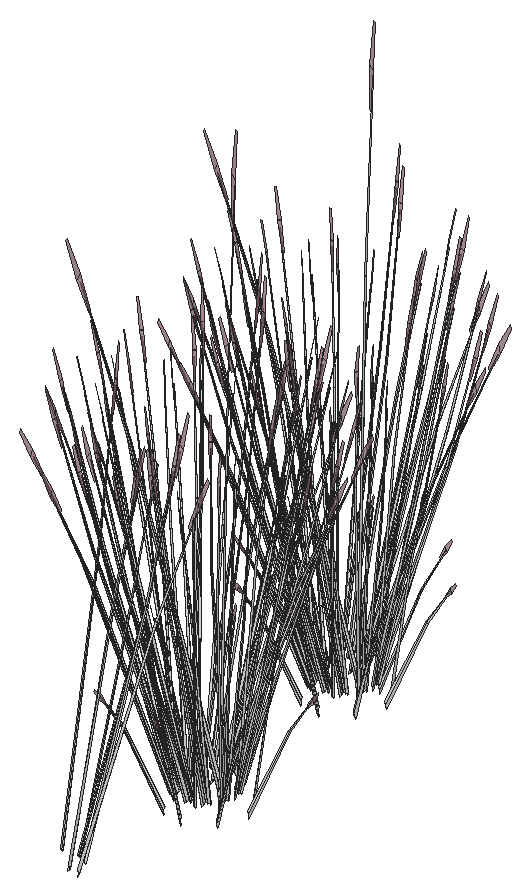
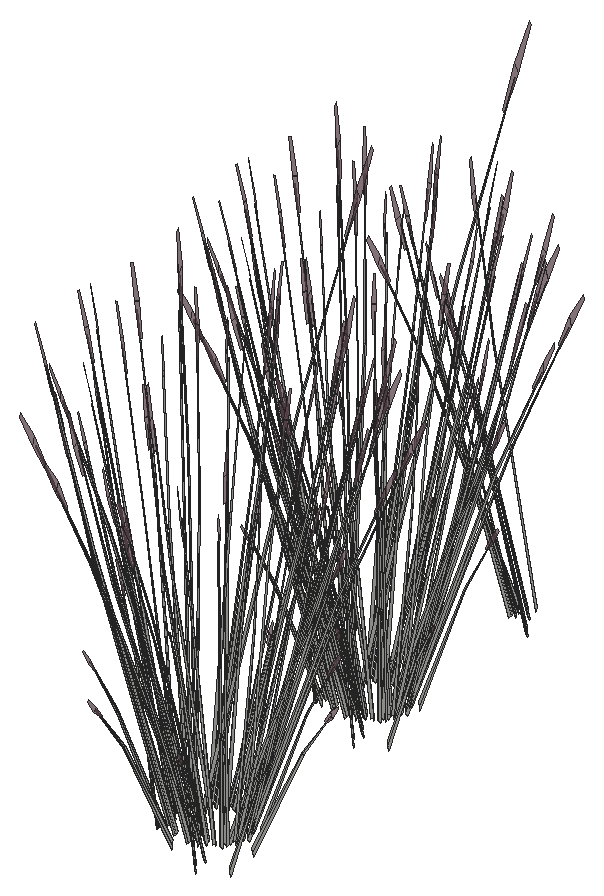
# SketchUp Ruby script. Lengths in inches.
U = 1.inch
M = Sketchup.active_model
def pt(a) = Geom::Point3d.new(a.map { |v| v * U })
def face(e, loops, mat)
  f = e.add_face(loops[0].map { |a| pt(a) })
  loops[1..].each { |l| e.add_face(l.map { |a| pt(a) }).erase! }
  f.material = f.back_material = mat if mat
  f
end
# faces: each face lists its corners as indices into pts; further lists are holes
def faces(e, pts, list, mat = nil) = list.each { |f| face(e, (f[0].is_a?(Array) ? f : [f]).map { |l| l.map { |i| pts[i] } }, mat) }
# xy, xz, yz: faces in a plane at the given z, y or x. An outline is a flat list of corners, or four numbers for a rectangle; further outlines are holes
def ring(l) = l.size == 4 ? [[l[0], l[1]], [l[2], l[1]], [l[2], l[3]], [l[0], l[3]]] : l.each_slice(2).to_a
def flat(e, list, mat, &to3) = list.each { |f| face(e, (f[0].is_a?(Array) ? f : [f]).map { |l| ring(l).map { |u, v| to3.(u, v) } }, mat) }
def xy(e, z, list, mat = nil) = flat(e, list, mat) { |x, y| [x, y, z] }
def xz(e, y, list, mat = nil) = flat(e, list, mat) { |x, z| [x, y, z] }
def yz(e, x, list, mat = nil) = flat(e, list, mat) { |y, z| [x, y, z] }
def lines(e, pts, list) = list.each { |a, b| e.add_line(pt(pts[a]), pt(pts[b])) }
# prism: a flat outline (further loops are holes) pulled along v
def prism(e, loops, v, mat = nil)
  f = face(e, loops, mat); d = Geom::Vector3d.new(v.map { |x| x * U })
  f.pushpull(f.normal.samedirection?(d) ? d.length : -d.length)
end
def box(e, o, s, mat = nil) = prism(e, [[o, [o[0] + s[0], o[1], o[2]], [o[0] + s[0], o[1] + s[1], o[2]], [o[0], o[1] + s[1], o[2]]]], [0, 0, s[2]], mat)
def at(x, y, z, deg = 0) = Geom::Transformation.translation(pt([x, y, z])) * Geom::Transformation.rotation(ORIGIN, Z_AXIS, deg.degrees)
def axes(o, x, y, z) = Geom::Transformation.new([*x, 0, *y, 0, *z, 0, *pt(o).to_a, 1])
def part(name) = M.definitions.add(name)
# library, detail: a bought-in or finely detailed component or shape, given as its bounding box
def library(name, o, s) = part(name).tap { |d| box(d.entities, o, s) }
def detail(e, o, s) = box(e.add_group.entities, o, s)
def put(e, d, t, mat = nil) = e.add_instance(d, t).tap { |i| i.material = mat if mat }
def group(e, t, mat = nil) = e.add_group.tap { |g| g.transformation = t; g.material = mat if mat }.entities
root = M.entities
M.materials.add("LightPink_Translucent").color = [144, 107, 117]
M.materials["LightPink_Translucent"].alpha = 0.75
c1 = part("blade")
p = [[2.15,0.21,22],[0,0.17,0],[0.09,0.45,0],[2.18,0.31,22],[2.29,0.31,22],[0.38,0.45,0],
  [2.48,0.24,33],[2.49,0.24,33],[2.48,0.22,33]]
faces(c1.entities,p,[[0,1,2,3],[4,5,2,3],[6,3,4,7],[8,0,3,6]])
c2 = part("seeds")
p = [[0.3,-0.1,1.38],[-0.01,-0.03,1.59],[-0.01,-0.03,0.03],[0.14,-0.07,-0.07],[0.29,-0.03,3],[0.15,0.01,3.11]]
faces(c2.entities,p,[[0,1,2,3],[1,0,4,5]],"LightPink_Translucent")
c3 = part("blade with seeds")
put(c3.entities,c1,at(0,0,0))
put(c3.entities,c2,axes([2.4,0.25,30.99],[1.5799,-0.05474,1.17369],[-0.12525,1.92788,0.29478],[-0.07173,-0.02425,1.56792]))
put(root,c3,axes([335.52,111.16,268.36],[0.50273,0.13626,-0.47583],[-0.17232,0.46717,-0.36857],[0.0461,0.18809,0.91046]))
put(root,c3,axes([335.81,110.19,267.61],[-0.1169,-0.17452,1.59586],[0.54019,-0.14692,0.12904],[0.12209,0.27397,0.68222]))
put(root,c3,axes([335.29,111.45,268.22],[-0.15418,0.41799,-0.32977],[-0.44981,-0.12192,0.42575],[0.04124,0.16829,0.81462]))
put(root,c3,axes([334.32,110.64,268.97],[-0.01331,0.50278,-0.73435],[-0.56035,-0.03377,0.08862],[-0.05914,0.213,1.03881]))
put(root,c3,axes([334.85,110.28,267.61],[-0.01252,-0.20862,1.59586],[0.54251,0.1384,0.12904],[-0.03356,0.2973,0.68222]))
put(root,c3,axes([335.34,111.07,268.64],[0.24409,0.44196,-0.66157],[-0.50245,0.2463,0.07984],[0.05708,0.21354,0.93586]))
put(root,c3,axes([334.13,111.35,267.13],[0.01124,-0.2806,1.43727],[0.50537,0.14821,0.19862],[-0.04379,0.29905,0.67868]))
put(root,c3,axes([334.52,122.62,267.61],[0.1169,0.17452,1.59586],[-0.54019,0.14692,0.12904],[-0.12209,-0.27397,0.68222]))
put(root,c3,axes([335.96,122.75,268.64],[-0.24409,-0.44196,-0.66157],[0.50245,-0.2463,0.07984],[-0.05708,-0.21354,0.93586]))
put(root,c3,axes([336.98,123.18,268.64],[0.01331,-0.50278,-0.66157],[0.56035,0.03377,0.07984],[0.05914,-0.213,0.93586]))
put(root,c3,axes([336.01,122.37,268.22],[0.15418,-0.41799,-0.32977],[0.44981,0.12192,0.42575],[-0.04124,-0.16829,0.81462]))
put(root,c3,axes([336.35,122.92,267.61],[-0.09522,0.18683,1.59586],[-0.39947,-0.38663,0.12904],[0.18021,-0.24097,0.68222]))
put(root,c3,axes([335.78,122.66,268.36],[-0.50273,-0.13626,-0.47583],[0.17232,-0.46717,-0.36857],[-0.0461,-0.18809,0.91046]))
put(root,c3,axes([336.09,121.49,266.58],[0.06561,0.31695,1.06958],[-0.36394,-0.17555,0.78586],[0.03916,-0.16229,0.23558]))
put(root,c3,axes([336.86,123.01,268.36],[-0.3661,-0.36521,-0.47583],[0.38674,-0.31985,-0.36857],[0.0557,-0.18556,0.91046]))
put(root,c3,axes([336.21,122.64,268.6875],[-0.50045,0.25306,-0.11324],[-0.24593,-0.44915,-0.62851],[-0.06603,-0.18927,0.95501]))
put(root,c3,axes([337.25,123.2,268.6875],[-0.56206,-0.02693,-0.11324],[0.01536,-0.50991,-0.62851],[0.03904,-0.19638,0.95501]))
put(root,c3,axes([337.21,122.88,268.22],[0.34603,-0.28618,-0.32977],[0.32756,0.32677,0.42575],[0.04984,-0.16603,0.81462]))
put(root,c3,axes([334.22,121.87,266.58],[0.26677,0.18918,1.06958],[-0.38851,0.11372,0.78586],[-0.08313,-0.14539,0.23558]))
put(root,c3,axes([334.86,122.87,268.64],[-0.43608,-0.26272,-0.66157],[0.30991,-0.46038,0.07984],[-0.158,-0.15687,0.93586]))
put(root,c3,axes([334.71,122.53,268.22],[-0.07899,-0.43781,-0.32977],[0.45153,-0.11561,0.42575],[-0.12128,-0.12546,0.81462]))
put(root,c3,axes([333.74,123.16,267.61],[0.18996,0.09365,1.59586],[-0.39312,0.39287,0.12904],[-0.24502,-0.17723,0.68222]))
put(root,c3,axes([334.66,122.89,268.36],[-0.50465,0.12921,-0.47583],[-0.08828,-0.48932,-0.36857],[-0.13555,-0.14022,0.91046]))
put(root,c3,axes([337.64,124.05,268.64],[0.26714,-0.42887,-0.66157],[0.46811,0.30479,0.07984],[0.1595,-0.15539,0.93586]))
put(root,c3,axes([337.625,123.85,268.36],[-0.13138,-0.49631,-0.47583],[0.49754,-0.08682,-0.36857],[0.14258,-0.13331,0.91046]))
put(root,c3,axes([337.86,124.21,268.6875],[-0.47307,-0.29971,-0.11324],[0.27254,-0.43404,-0.62851],[0.13365,-0.15087,0.95501]))
put(root,c3,axes([335.91,125.85,267.1],[0.44194,0.21918,1.40854],[-0.43295,0.47219,0.557],[-0.19393,-0.27986,1.18082]))
put(root,c3,axes([338.24,122.87,266.58],[-0.17034,0.27669,1.06958],[-0.14642,-0.37174,0.78586],[0.14069,-0.09315,0.23558]))
put(root,c3,axes([337.99,123.91,268.22],[0.44516,-0.07768,-0.32977],[0.11755,0.44407,0.42575],[0.12757,-0.11927,0.81462]))
put(root,c3,axes([333.67,123.3,268.22],[-0.29098,-0.34031,-0.32977],[0.33226,-0.32215,0.42575],[-0.16881,-0.04902,0.81462]))
put(root,c3,axes([333.97,123.52,268.64],[-0.51122,-0.01309,-0.66157],[0.03434,-0.5511,0.07984],[-0.21658,-0.05816,0.93586]))
put(root,c3,axes([333.8,123.63,268.36],[-0.37135,0.36005,-0.47583],[-0.32522,-0.38035,-0.36857],[-0.18868,-0.05478,0.91046]))
put(root,c3,axes([334,123.26,268.6875],[-0.02738,0.55277,-0.11324],[-0.51847,-0.01511,-0.62851],[-0.19968,-0.0384,0.95501]))
put(root,c3,axes([337.88,125.38,268.6875],[-0.25732,-0.49218,-0.11324],[0.45669,-0.24187,-0.62851],[0.19245,-0.06494,0.95501]))
put(root,c3,axes([337.86,124.96,268.36],[0.13855,-0.49442,-0.47583],[0.47502,0.16947,-0.36857],[0.19125,-0.04534,0.91046]))
put(root,c3,axes([333.34,124.02,267.61],[0.21212,-0.01231,1.59586],[-0.14072,0.53355,0.12904],[-0.3023,-0.033,0.68222]))
put(root,c3,axes([337.77,125.14,268.64],[0.44939,-0.24006,-0.66157],[0.25044,0.49415,0.07984],[0.21713,-0.05613,0.93586]))
put(root,c3,axes([338.15,125.18,268.22],[0.42502,0.15163,-0.32977],[-0.12396,0.44238,0.42575],[0.17112,-0.04056,0.81462]))
put(root,c3,axes([333.15,124.48,268.22],[-0.42502,-0.15163,-0.32977],[0.12396,-0.44238,0.42575],[-0.17112,0.04056,0.81462]))
put(root,c3,axes([336.99,124.63,267.61],[-0.21212,0.01231,1.59586],[0.14072,-0.53355,0.12904],[0.3023,0.033,0.68222]))
put(root,c3,axes([334.45,124.4,267.11],[0.14537,-0.07863,1.64882],[0.05013,0.549,0.12904],[-0.31487,0.07285,0.5893]))
put(root,c3,axes([339.05,125.27,266.58],[-0.31598,0.08973,1.06958],[0.14873,-0.37085,0.78586],[0.16763,0.02538,0.23558]))
put(root,c3,axes([333.44,124.7,268.36],[-0.13855,0.49442,-0.47583],[-0.47502,-0.16947,-0.36857],[-0.19125,0.04534,0.91046]))
put(root,c3,axes([333.42,124.28,268.6875],[0.25732,0.49218,-0.11324],[-0.45669,0.24187,-0.62851],[-0.19245,0.06494,0.95501]))
put(root,c3,axes([338.5,126.41,267.66],[-0.09788,-0.45691,-0.03251],[0.46264,-0.10504,-0.14742],[0.09661,0.02897,0.48626]))
put(root,c3,axes([337.3,126.4,268.6875],[0.02738,-0.55277,-0.11324],[0.51847,0.01511,-0.62851],[0.19968,0.0384,0.95501]))
put(root,c3,axes([333.43,124.96,267.61],[0.17745,-0.11497,1.59586],[0.14939,0.53127,0.12904],[-0.27857,0.12007,0.68222]))
put(root,c3,axes([337.33,126.14,268.64],[0.51122,0.01309,-0.66157],[-0.03434,0.5511,0.07984],[0.21658,0.05816,0.93586]))
put(root,c3,axes([332.5,126.82,266.58],[0.21313,-0.24635,1.06958],[0.0841,0.38999,0.78586],[-0.15402,0.06983,0.23558]))
put(root,c3,axes([337.63,126.36,268.22],[0.29098,0.34031,-0.32977],[-0.33226,0.32215,0.42575],[0.16881,0.04902,0.81462]))
put(root,c3,axes([333.31,125.75,268.22],[-0.44516,0.07768,-0.32977],[-0.11755,-0.44407,0.42575],[-0.12757,0.11927,0.81462]))
put(root,c3,axes([336.59,125.49,267.61],[-0.18996,-0.09365,1.59586],[0.39312,-0.39287,0.12904],[0.24502,0.17723,0.68222]))
put(root,c3,axes([333.44,125.45,268.6875],[0.47307,0.29971,-0.11324],[-0.27254,0.43404,-0.62851],[-0.13365,0.15087,0.95501]))
put(root,c3,axes([336.28,127,268.6875],[0.30474,-0.46525,-0.11324],[0.44133,0.26804,-0.62851],[0.15341,0.13145,0.95501]))
put(root,c3,axes([334.08,125.31,267.61],[0.12773,-0.16701,1.59586],[0.32252,0.4508,0.12904],[-0.22121,0.20529,0.68222]))
put(root,c3,axes([333.67,125.8,268.36],[0.13138,0.49631,-0.47583],[-0.49754,0.08682,-0.36857],[-0.14258,0.13331,0.91046]))
put(root,c3,axes([336.59,124.8,266.65],[-0.01397,-0.51177,1.31553],[0.63227,0.13266,0.557],[-0.14954,0.28003,1.24175]))
put(root,c3,axes([336.64,126.77,268.36],[0.50465,-0.12921,-0.47583],[0.08828,0.48932,-0.36857],[0.13555,0.14022,0.91046]))
put(root,c3,axes([333.98,125.73,267.61],[0.09522,-0.18683,1.59586],[0.39947,0.38663,0.12904],[-0.18021,0.24097,0.68222]))
put(root,c3,axes([334.09,126.78,268.22],[-0.34603,0.28618,-0.32977],[-0.32756,-0.32677,0.42575],[-0.04984,0.16603,0.81462]))
put(root,c3,axes([335.09,127.02,268.6875],[0.50045,-0.25306,-0.11324],[0.24593,0.44915,-0.62851],[0.06603,0.18927,0.95501]))
put(root,c3,axes([334.3125,127.89,266.58],[-0.01324,-0.32319,1.06958],[0.33072,0.23052,0.78586],[-0.06504,0.15405,0.23558]))
put(root,c3,axes([334.43,126.64,268.66],[0.3661,0.36521,-0.52818],[-0.38674,0.31985,-0.40911],[-0.0557,0.18556,1.01061]))
put(root,c3,axes([335.52,127,268.36],[0.50273,0.13626,-0.47583],[-0.17232,0.46717,-0.36857],[0.0461,0.18809,0.91046]))
put(root,c3,axes([335.81,126.03,267.61],[-0.1169,-0.17452,1.59586],[0.54019,-0.14692,0.12904],[0.12209,0.27397,0.68222]))
put(root,c3,axes([335.29,127.29,268.22],[-0.15418,0.41799,-0.32977],[-0.44981,-0.12192,0.42575],[0.04124,0.16829,0.81462]))
put(root,c3,axes([334.32,126.48,268.97],[-0.01331,0.50278,-0.73435],[-0.56035,-0.03377,0.08862],[-0.05914,0.213,1.03881]))
put(root,c3,axes([334.85,126.12,267.61],[-0.01252,-0.20862,1.59586],[0.54251,0.1384,0.12904],[-0.03356,0.2973,0.68222]))
put(root,c3,axes([335.34,126.91,268.64],[0.24409,0.44196,-0.66157],[-0.50245,0.2463,0.07984],[0.05708,0.21354,0.93586]))
put(root,c3,axes([334.13,127.1875,267.13],[0.01124,-0.2806,1.43727],[0.50537,0.14821,0.19862],[-0.04379,0.29905,0.67868]))
put(root,c3,axes([332.31,140.63,267.61],[0.1169,0.17452,1.59586],[-0.54019,0.14692,0.12904],[-0.12209,-0.27397,0.68222]))
put(root,c3,axes([333.75,140.76,268.64],[-0.24409,-0.44196,-0.66157],[0.50245,-0.2463,0.07984],[-0.05708,-0.21354,0.93586]))
put(root,c3,axes([334.76,141.19,268.64],[0.01331,-0.50278,-0.66157],[0.56035,0.03377,0.07984],[0.05914,-0.213,0.93586]))
put(root,c3,axes([333.79,140.38,268.22],[0.15418,-0.41799,-0.32977],[0.44981,0.12192,0.42575],[-0.04124,-0.16829,0.81462]))
put(root,c3,axes([334.13,140.93,267.61],[-0.09522,0.18683,1.59586],[-0.39947,-0.38663,0.12904],[0.18021,-0.24097,0.68222]))
put(root,c3,axes([333.5625,140.67,268.36],[-0.50273,-0.13626,-0.47583],[0.17232,-0.46717,-0.36857],[-0.0461,-0.18809,0.91046]))
put(root,c3,axes([333.875,139.5,266.58],[0.06561,0.31695,1.06958],[-0.36394,-0.17555,0.78586],[0.03916,-0.16229,0.23558]))
put(root,c3,axes([334.65,141.02,268.36],[-0.3661,-0.36521,-0.47583],[0.38674,-0.31985,-0.36857],[0.0557,-0.18556,0.91046]))
put(root,c3,axes([335.03,141.21,268.6875],[-0.56206,-0.02693,-0.11324],[0.01536,-0.50991,-0.62851],[0.03904,-0.19638,0.95501]))
put(root,c3,axes([334.99,140.89,268.22],[0.34603,-0.28618,-0.32977],[0.32756,0.32677,0.42575],[0.04984,-0.16603,0.81462]))
put(root,c3,axes([332,139.88,266.58],[0.26677,0.18918,1.06958],[-0.38851,0.11372,0.78586],[-0.08313,-0.14539,0.23558]))
put(root,c3,axes([332.65,140.88,268.64],[-0.43608,-0.26272,-0.66157],[0.30991,-0.46038,0.07984],[-0.158,-0.15687,0.93586]))
put(root,c3,axes([332.5,140.53,268.22],[-0.07899,-0.43781,-0.32977],[0.45153,-0.11561,0.42575],[-0.12128,-0.12546,0.81462]))
put(root,c3,axes([331.52,141.17,267.61],[0.18996,0.09365,1.59586],[-0.39312,0.39287,0.12904],[-0.24502,-0.17723,0.68222]))
put(root,c3,axes([332.44,140.9,268.36],[-0.50465,0.12921,-0.47583],[-0.08828,-0.48932,-0.36857],[-0.13555,-0.14022,0.91046]))
put(root,c3,axes([335.42,142.0625,268.64],[0.26714,-0.42887,-0.66157],[0.46811,0.30479,0.07984],[0.1595,-0.15539,0.93586]))
put(root,c3,axes([335.41,141.86,268.36],[-0.13138,-0.49631,-0.47583],[0.49754,-0.08682,-0.36857],[0.14258,-0.13331,0.91046]))
put(root,c3,axes([333.69,143.85,267.1],[0.44194,0.21918,1.40854],[-0.43295,0.47219,0.557],[-0.19393,-0.27986,1.18082]))
put(root,c3,axes([336.02,140.875,266.58],[-0.17034,0.27669,1.06958],[-0.14642,-0.37174,0.78586],[0.14069,-0.09315,0.23558]))
put(root,c3,axes([335.78,141.92,268.22],[0.44516,-0.07768,-0.32977],[0.11755,0.44407,0.42575],[0.12757,-0.11927,0.81462]))
put(root,c3,axes([331.45,141.31,268.22],[-0.29098,-0.34031,-0.32977],[0.33226,-0.32215,0.42575],[-0.16881,-0.04902,0.81462]))
put(root,c3,axes([331.76,141.53,268.64],[-0.51122,-0.01309,-0.66157],[0.03434,-0.5511,0.07984],[-0.21658,-0.05816,0.93586]))
put(root,c3,axes([331.59,141.64,268.36],[-0.37135,0.36005,-0.47583],[-0.32522,-0.38035,-0.36857],[-0.18868,-0.05478,0.91046]))
put(root,c3,axes([330.75,142.12,266.58],[0.3265,-0.03889,1.06958],[-0.20711,0.3427,0.78586],[-0.16135,-0.05141,0.23558]))
put(root,c3,axes([331.78,141.27,268.6875],[-0.02738,0.55277,-0.11324],[-0.51847,-0.01511,-0.62851],[-0.19968,-0.0384,0.95501]))
put(root,c3,axes([335.66,143.39,268.6875],[-0.25732,-0.49218,-0.11324],[0.45669,-0.24187,-0.62851],[0.19245,-0.06494,0.95501]))
put(root,c3,axes([335.64,142.97,268.36],[0.13855,-0.49442,-0.47583],[0.47502,0.16947,-0.36857],[0.19125,-0.04534,0.91046]))
put(root,c3,axes([331.125,142.03,267.61],[0.21212,-0.01231,1.59586],[-0.14072,0.53355,0.12904],[-0.3023,-0.033,0.68222]))
put(root,c3,axes([335.55,143.15,268.64],[0.44939,-0.24006,-0.66157],[0.25044,0.49415,0.07984],[0.21713,-0.05613,0.93586]))
put(root,c3,axes([335.93,143.19,268.22],[0.42502,0.15163,-0.32977],[-0.12396,0.44238,0.42575],[0.17112,-0.04056,0.81462]))
put(root,c3,axes([330.9375,142.49,268.22],[-0.42502,-0.15163,-0.32977],[0.12396,-0.44238,0.42575],[-0.17112,0.04056,0.81462]))
put(root,c3,axes([334.77,142.64,267.61],[-0.21212,0.01231,1.59586],[0.14072,-0.53355,0.12904],[0.3023,0.033,0.68222]))
put(root,c3,axes([332.23,142.41,267.11],[0.14537,-0.07863,1.64882],[0.05013,0.549,0.12904],[-0.31487,0.07285,0.5893]))
put(root,c3,axes([336.83,143.28,266.58],[-0.31598,0.08973,1.06958],[0.14873,-0.37085,0.78586],[0.16763,0.02538,0.23558]))
put(root,c3,axes([331.23,142.71,268.36],[-0.13855,0.49442,-0.47583],[-0.47502,-0.16947,-0.36857],[-0.19125,0.04534,0.91046]))
put(root,c3,axes([331.21,142.29,268.6875],[0.25732,0.49218,-0.11324],[-0.45669,0.24187,-0.62851],[-0.19245,0.06494,0.95501]))
put(root,c3,axes([336.28,144.42,267.66],[-0.09788,-0.45691,-0.03251],[0.46264,-0.10504,-0.14742],[0.09661,0.02897,0.48626]))
put(root,c3,axes([335.09,144.41,268.6875],[0.02738,-0.55277,-0.11324],[0.51847,0.01511,-0.62851],[0.19968,0.0384,0.95501]))
put(root,c3,axes([331.21,142.97,267.61],[0.17745,-0.11497,1.59586],[0.14939,0.53127,0.12904],[-0.27857,0.12007,0.68222]))
put(root,c3,axes([335.11,144.14,268.64],[0.51122,0.01309,-0.66157],[-0.03434,0.5511,0.07984],[0.21658,0.05816,0.93586]))
put(root,c3,axes([330.29,144.83,266.58],[0.21313,-0.24635,1.06958],[0.0841,0.38999,0.78586],[-0.15402,0.06983,0.23558]))
put(root,c3,axes([335.42,144.37,268.22],[0.29098,0.34031,-0.32977],[-0.33226,0.32215,0.42575],[0.16881,0.04902,0.81462]))
put(root,c3,axes([331.09,143.76,268.22],[-0.44516,0.07768,-0.32977],[-0.11755,-0.44407,0.42575],[-0.12757,0.11927,0.81462]))
put(root,c3,axes([334.37,143.5,267.61],[-0.18996,-0.09365,1.59586],[0.39312,-0.39287,0.12904],[0.24502,0.17723,0.68222]))
put(root,c3,axes([335.08,144.57,266.58],[-0.28795,-0.15629,1.06958],[0.37181,-0.1588,0.78586],[0.10029,0.13452,0.23558]))
put(root,c3,axes([331.86,143.32,267.61],[0.12773,-0.16701,1.59586],[0.32252,0.4508,0.12904],[-0.22121,0.20529,0.68222]))
put(root,c3,axes([331.46,143.8125,268.36],[0.13138,0.49631,-0.47583],[-0.49754,0.08682,-0.36857],[-0.14258,0.13331,0.91046]))
put(root,c3,axes([334.375,142.81,266.65],[-0.01397,-0.51177,1.31553],[0.63227,0.13266,0.557],[-0.14954,0.28003,1.24175]))
put(root,c3,axes([334.43,144.78,268.36],[0.50465,-0.12921,-0.47583],[0.08828,0.48932,-0.36857],[0.13555,0.14022,0.91046]))
put(root,c3,axes([331.76,143.74,267.61],[0.09522,-0.18683,1.59586],[0.39947,0.38663,0.12904],[-0.18021,0.24097,0.68222]))
put(root,c3,axes([331.875,144.79,268.22],[-0.34603,0.28618,-0.32977],[-0.32756,-0.32677,0.42575],[-0.04984,0.16603,0.81462]))
put(root,c3,axes([332.875,145.03,268.6875],[0.50045,-0.25306,-0.11324],[0.24593,0.44915,-0.62851],[0.06603,0.18927,0.95501]))
put(root,c3,axes([332.1,145.9,266.58],[-0.01324,-0.32319,1.06958],[0.33072,0.23052,0.78586],[-0.06504,0.15405,0.23558]))
put(root,c3,axes([332.22,144.65,268.66],[0.3661,0.36521,-0.52818],[-0.38674,0.31985,-0.40911],[-0.0557,0.18556,1.01061]))
put(root,c3,axes([333.31,145.01,268.36],[0.50273,0.13626,-0.47583],[-0.17232,0.46717,-0.36857],[0.0461,0.18809,0.91046]))
put(root,c3,axes([333.59,144.04,267.61],[-0.1169,-0.17452,1.59586],[0.54019,-0.14692,0.12904],[0.12209,0.27397,0.68222]))
put(root,c3,axes([333.08,145.3,268.22],[-0.15418,0.41799,-0.32977],[-0.44981,-0.12192,0.42575],[0.04124,0.16829,0.81462]))
put(root,c3,axes([332.11,144.49,268.97],[-0.01331,0.50278,-0.73435],[-0.56035,-0.03377,0.08862],[-0.05914,0.213,1.03881]))
put(root,c3,axes([332.64,144.13,267.61],[-0.01252,-0.20862,1.59586],[0.54251,0.1384,0.12904],[-0.03356,0.2973,0.68222]))
put(root,c3,axes([333.12,144.92,268.64],[0.24409,0.44196,-0.66157],[-0.50245,0.2463,0.07984],[0.05708,0.21354,0.93586]))
put(root,c3,axes([331.92,145.2,267.13],[0.01124,-0.2806,1.43727],[0.50537,0.14821,0.19862],[-0.04379,0.29905,0.67868]))
